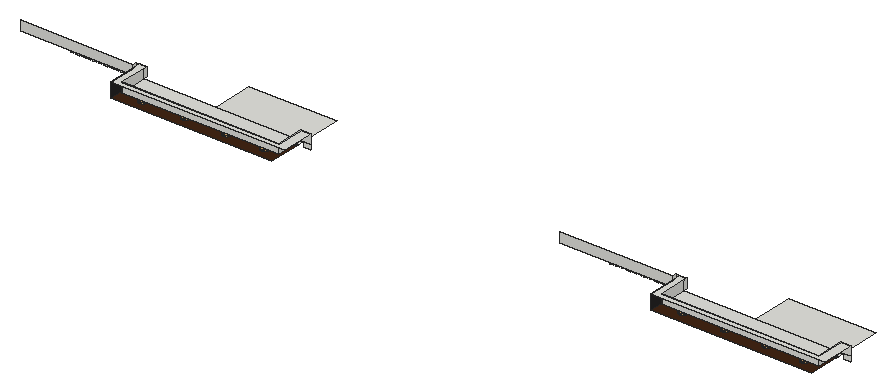
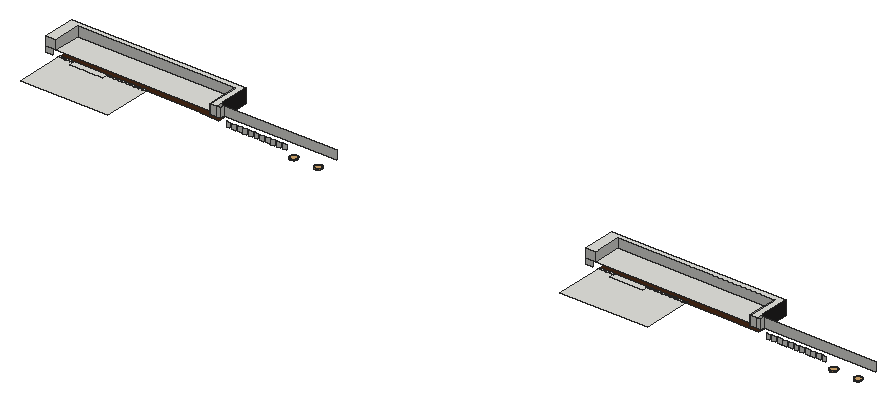
# SketchUp Ruby script. Lengths in inches.
U = 1.inch
M = Sketchup.active_model
def pt(a) = Geom::Point3d.new(a.map { |v| v * U })
def face(e, loops, mat)
  f = e.add_face(loops[0].map { |a| pt(a) })
  loops[1..].each { |l| e.add_face(l.map { |a| pt(a) }).erase! }
  f.material = f.back_material = mat if mat
  f
end
# faces: each face lists its corners as indices into pts; further lists are holes
def faces(e, pts, list, mat = nil) = list.each { |f| face(e, (f[0].is_a?(Array) ? f : [f]).map { |l| l.map { |i| pts[i] } }, mat) }
# xy, xz, yz: faces in a plane at the given z, y or x. An outline is a flat list of corners, or four numbers for a rectangle; further outlines are holes
def ring(l) = l.size == 4 ? [[l[0], l[1]], [l[2], l[1]], [l[2], l[3]], [l[0], l[3]]] : l.each_slice(2).to_a
def flat(e, list, mat, &to3) = list.each { |f| face(e, (f[0].is_a?(Array) ? f : [f]).map { |l| ring(l).map { |u, v| to3.(u, v) } }, mat) }
def xy(e, z, list, mat = nil) = flat(e, list, mat) { |x, y| [x, y, z] }
def xz(e, y, list, mat = nil) = flat(e, list, mat) { |x, z| [x, y, z] }
def yz(e, x, list, mat = nil) = flat(e, list, mat) { |y, z| [x, y, z] }
def lines(e, pts, list) = list.each { |a, b| e.add_line(pt(pts[a]), pt(pts[b])) }
# prism: a flat outline (further loops are holes) pulled along v
def prism(e, loops, v, mat = nil)
  f = face(e, loops, mat); d = Geom::Vector3d.new(v.map { |x| x * U })
  f.pushpull(f.normal.samedirection?(d) ? d.length : -d.length)
end
def box(e, o, s, mat = nil) = prism(e, [[o, [o[0] + s[0], o[1], o[2]], [o[0] + s[0], o[1] + s[1], o[2]], [o[0], o[1] + s[1], o[2]]]], [0, 0, s[2]], mat)
def at(x, y, z, deg = 0) = Geom::Transformation.translation(pt([x, y, z])) * Geom::Transformation.rotation(ORIGIN, Z_AXIS, deg.degrees)
def axes(o, x, y, z) = Geom::Transformation.new([*x, 0, *y, 0, *z, 0, *pt(o).to_a, 1])
def part(name) = M.definitions.add(name)
# library, detail: a bought-in or finely detailed component or shape, given as its bounding box
def library(name, o, s) = part(name).tap { |d| box(d.entities, o, s) }
def detail(e, o, s) = box(e.add_group.entities, o, s)
def put(e, d, t, mat = nil) = e.add_instance(d, t).tap { |i| i.material = mat if mat }
def group(e, t, mat = nil) = e.add_group.tap { |g| g.transformation = t; g.material = mat if mat }.entities
root = M.entities
M.materials.add("[Field Square Tile]").color = [211, 167, 108]
M.materials.add("[Granite Dark Gray]").color = [38, 37, 37]
M.materials.add("[Wood Veneer 01]").color = [66, 38, 20]
xy(root,380.5,[[534.46,508.33,539.88,511.08],[539.88,508.33,541.08,511.08],[541.08,508.33,546.51,511.08],[546.51,508.33,547.71,511.08],[547.71,508.33,553.13,511.08],
  [553.13,508.33,554.33,511.08],[554.33,508.33,559.76,511.08],[559.76,508.33,560.96,511.08],[560.96,508.33,566.38,511.08],[566.38,508.33,567.58,511.08],
  [567.58,508.33,573.01,511.08],[573.01,508.33,574.21,511.08],[574.21,508.33,579.63,511.08],[579.63,508.33,580.83,511.08],[580.83,508.33,586.26,511.08],
  [586.26,508.33,587.46,511.08],[587.46,508.33,592.88,511.08],[592.88,508.33,594.08,511.08],[594.08,508.33,599.51,511.08],[599.51,508.33,653.06,518.65],
  [653.06,508.33,658.48,511.08],[658.48,508.33,659.68,511.08],[659.68,508.33,665.11,511.08],[665.11,508.33,666.31,511.08],[666.31,508.33,671.73,511.08],
  [671.73,508.33,672.56,511.08],[672.56,508.33,676.54,511.08],[676.54,508.33,677.98,511.08],[1413.21,508.33,1418.63,511.08],[1418.63,508.33,1419.83,511.08],
  [1419.83,508.33,1425.26,511.08],[1425.26,508.33,1426.46,511.08],[1426.46,508.33,1431.88,511.08],[1431.88,508.33,1433.08,511.08],[1433.08,508.33,1438.51,511.08],
  [1438.51,508.33,1439.71,511.08],[1439.71,508.33,1445.13,511.08],[1445.13,508.33,1446.33,511.08],[1446.33,508.33,1451.76,511.08],[1451.76,508.33,1452.96,511.08],
  [1452.96,508.33,1458.38,511.08],[1458.38,508.33,1459.58,511.08],[1459.58,508.33,1465.01,511.08],[1465.01,508.33,1466.21,511.08],[1466.21,508.33,1471.63,511.08],
  [1471.63,508.33,1472.83,511.08],[1472.83,508.33,1478.26,511.08],[1478.26,508.33,1531.81,518.65],[1531.81,508.33,1537.23,511.08],[1537.23,508.33,1538.43,511.08],
  [1538.43,508.33,1543.86,511.08],[1543.86,508.33,1545.06,511.08],[1545.06,508.33,1550.48,511.08],[1550.48,508.33,1551.31,511.08],[1551.31,508.33,1555.29,511.08],
  [1555.29,508.33,1556.73,511.08],[534.46,511.08,534.46,589.83,676.54,589.83,676.54,511.08,653.06,511.08,653.06,518.65,599.51,518.65,599.51,511.08],[1413.21,511.08,1413.21,589.83,1555.29,589.83,1555.29,511.08,1531.81,511.08,1531.81,518.65,1478.26,518.65,1478.26,511.08]])
xy(root,380.5,[[[414.98,458.5,414.98,512.27,444.78,512.27,444.78,511.08,534.46,511.08,534.46,508.33,676.54,508.33,676.54,458.5],[521.68,470.7,523.23,470.9,524.68,471.5,525.92,472.46,526.88,473.7,527.48,475.15,527.68,476.7,527.48,478.25,526.88,479.7,525.92,480.94,524.68,481.9,523.23,482.49,521.68,482.7,520.13,482.49,518.68,481.9,517.4375,480.94,516.49,479.7,515.89,478.25,515.68,476.7,515.89,475.15,516.49,473.7,517.4375,472.46,518.68,471.5,520.13,470.9],[588.96,470.7,590.51,470.9,591.96,471.5,593.2,472.46,594.16,473.7,594.76,475.15,594.96,476.7,594.76,478.25,594.16,479.7,593.2,480.94,591.96,481.9,590.51,482.49,588.96,482.7,587.41,482.49,585.96,481.9,584.72,480.94,583.76,479.7,583.16,478.25,582.96,476.7,583.16,475.15,583.76,473.7,584.72,472.46,585.96,471.5,587.41,470.9],[650.33,470.7,651.89,470.9,653.33,471.5,654.58,472.46,655.53,473.7,656.13,475.15,656.33,476.7,656.13,478.25,655.53,479.7,654.58,480.94,653.33,481.9,651.89,482.49,650.33,482.7,648.78,482.49,647.33,481.9,646.09,480.94,645.14,479.7,644.54,478.25,644.33,476.7,644.54,475.15,645.14,473.7,646.09,472.46,647.33,471.5,648.78,470.9],[452.22,470.7,453.77,470.9,455.22,471.5,456.46,472.46,457.41,473.7,458.01,475.15,458.22,476.7,458.01,478.25,457.41,479.7,456.46,480.94,455.22,481.9,453.77,482.49,452.22,482.7,450.67,482.49,449.22,481.9,447.98,480.94,447.02,479.7,446.42,478.25,446.22,476.7,446.42,475.15,447.02,473.7,447.98,472.46,449.22,471.5,450.67,470.9]],[[1293.73,458.5,1293.73,512.27,1323.53,512.27,1323.53,511.08,1413.21,511.08,1413.21,508.33,1555.29,508.33,1555.29,458.5],[1400.43,470.7,1401.98,470.9,1403.43,471.5,1404.67,472.46,1405.63,473.7,1406.23,475.15,1406.43,476.7,1406.23,478.25,1405.63,479.7,1404.67,480.94,1403.43,481.9,1401.98,482.49,1400.43,482.7,1398.88,482.49,1397.43,481.9,1396.1875,480.94,1395.24,479.7,1394.64,478.25,1394.43,476.7,1394.64,475.15,1395.24,473.7,1396.1875,472.46,1397.43,471.5,1398.88,470.9],[1529.08,470.7,1530.64,470.9,1532.08,471.5,1533.33,472.46,1534.28,473.7,1534.88,475.15,1535.08,476.7,1534.88,478.25,1534.28,479.7,1533.33,480.94,1532.08,481.9,1530.64,482.49,1529.08,482.7,1527.53,482.49,1526.08,481.9,1524.84,480.94,1523.89,479.7,1523.29,478.25,1523.08,476.7,1523.29,475.15,1523.89,473.7,1524.84,472.46,1526.08,471.5,1527.53,470.9],[1330.97,470.7,1332.52,470.9,1333.97,471.5,1335.21,472.46,1336.16,473.7,1336.76,475.15,1336.97,476.7,1336.76,478.25,1336.16,479.7,1335.21,480.94,1333.97,481.9,1332.52,482.49,1330.97,482.7,1329.42,482.49,1327.97,481.9,1326.73,480.94,1325.77,479.7,1325.17,478.25,1324.97,476.7,1325.17,475.15,1325.77,473.7,1326.73,472.46,1327.97,471.5,1329.42,470.9],[1467.71,470.7,1469.26,470.9,1470.71,471.5,1471.95,472.46,1472.91,473.7,1473.51,475.15,1473.71,476.7,1473.51,478.25,1472.91,479.7,1471.95,480.94,1470.71,481.9,1469.26,482.49,1467.71,482.7,1466.16,482.49,1464.71,481.9,1463.47,480.94,1462.51,479.7,1461.91,478.25,1461.71,476.7,1461.91,475.15,1462.51,473.7,1463.47,472.46,1464.71,471.5,1466.16,470.9]]],"[Wood Veneer 01]")
xy(root,381.8125,[[452.22,470.7,450.67,470.9,449.22,471.5,447.98,472.46,447.02,473.7,446.42,475.15,446.22,476.7,446.42,478.25,447.02,479.7,447.98,480.94,449.22,481.9,450.67,482.49,452.22,482.7,453.77,482.49,455.22,481.9,456.46,480.94,457.41,479.7,458.01,478.25,458.22,476.7,458.01,475.15,457.41,473.7,456.46,472.46,455.22,471.5,453.77,470.9],[521.68,470.7,520.13,470.9,518.68,471.5,517.4375,472.46,516.49,473.7,515.89,475.15,515.68,476.7,515.89,478.25,516.49,479.7,517.4375,480.94,518.68,481.9,520.13,482.49,521.68,482.7,523.23,482.49,524.68,481.9,525.92,480.94,526.88,479.7,527.48,478.25,527.68,476.7,527.48,475.15,526.88,473.7,525.92,472.46,524.68,471.5,523.23,470.9],[588.96,470.7,587.41,470.9,585.96,471.5,584.72,472.46,583.76,473.7,583.16,475.15,582.96,476.7,583.16,478.25,583.76,479.7,584.72,480.94,585.96,481.9,587.41,482.49,588.96,482.7,590.51,482.49,591.96,481.9,593.2,480.94,594.16,479.7,594.76,478.25,594.96,476.7,594.76,475.15,594.16,473.7,593.2,472.46,591.96,471.5,590.51,470.9],[650.33,470.7,648.78,470.9,647.33,471.5,646.09,472.46,645.14,473.7,644.54,475.15,644.33,476.7,644.54,478.25,645.14,479.7,646.09,480.94,647.33,481.9,648.78,482.49,650.33,482.7,651.89,482.49,653.33,481.9,654.58,480.94,655.53,479.7,656.13,478.25,656.33,476.7,656.13,475.15,655.53,473.7,654.58,472.46,653.33,471.5,651.89,470.9],[1330.97,470.7,1329.42,470.9,1327.97,471.5,1326.73,472.46,1325.77,473.7,1325.17,475.15,1324.97,476.7,1325.17,478.25,1325.77,479.7,1326.73,480.94,1327.97,481.9,1329.42,482.49,1330.97,482.7,1332.52,482.49,1333.97,481.9,1335.21,480.94,1336.16,479.7,1336.76,478.25,1336.97,476.7,1336.76,475.15,1336.16,473.7,1335.21,472.46,1333.97,471.5,1332.52,470.9],
  [1400.43,470.7,1398.88,470.9,1397.43,471.5,1396.1875,472.46,1395.24,473.7,1394.64,475.15,1394.43,476.7,1394.64,478.25,1395.24,479.7,1396.1875,480.94,1397.43,481.9,1398.88,482.49,1400.43,482.7,1401.98,482.49,1403.43,481.9,1404.67,480.94,1405.63,479.7,1406.23,478.25,1406.43,476.7,1406.23,475.15,1405.63,473.7,1404.67,472.46,1403.43,471.5,1401.98,470.9],[1467.71,470.7,1466.16,470.9,1464.71,471.5,1463.47,472.46,1462.51,473.7,1461.91,475.15,1461.71,476.7,1461.91,478.25,1462.51,479.7,1463.47,480.94,1464.71,481.9,1466.16,482.49,1467.71,482.7,1469.26,482.49,1470.71,481.9,1471.95,480.94,1472.91,479.7,1473.51,478.25,1473.71,476.7,1473.51,475.15,1472.91,473.7,1471.95,472.46,1470.71,471.5,1469.26,470.9],[1529.08,470.7,1527.53,470.9,1526.08,471.5,1524.84,472.46,1523.89,473.7,1523.29,475.15,1523.08,476.7,1523.29,478.25,1523.89,479.7,1524.84,480.94,1526.08,481.9,1527.53,482.49,1529.08,482.7,1530.64,482.49,1532.08,481.9,1533.33,480.94,1534.28,479.7,1534.88,478.25,1535.08,476.7,1534.88,475.15,1534.28,473.7,1533.33,472.46,1532.08,471.5,1530.64,470.9]],"[Field Square Tile]")
xy(root,381.875,[[240.83,523.51,239.27,523.54,237.76,523.98,236.42,524.79,235.34,525.92,234.58,527.29,234.21,528.8125,234.24,530.375,234.68,531.88,235.49,533.22,236.62,534.31,237.99,535.06,239.51,535.43,241.08,535.4,242.58,534.96,243.92,534.15,245.01,533.02,245.76,531.65,246.14,530.13,246.1,528.5625,245.67,527.06,244.86,525.72,243.73,524.64,242.35,523.88],[280.58,523.51,279.02,523.54,277.51,523.98,276.17,524.79,275.09,525.92,274.33,527.29,273.96,528.8125,273.99,530.375,274.43,531.88,275.24,533.22,276.37,534.31,277.74,535.06,279.26,535.43,280.83,535.4,282.33,534.96,283.67,534.15,284.76,533.02,285.51,531.65,285.89,530.13,285.85,528.5625,285.42,527.06,284.61,525.72,283.48,524.64,282.1,523.88],[1119.58,523.51,1118.02,523.54,1116.51,523.98,1115.17,524.79,1114.09,525.92,1113.33,527.29,1112.96,528.8125,1112.99,530.375,1113.43,531.88,1114.24,533.22,1115.37,534.31,1116.74,535.06,1118.26,535.43,1119.83,535.4,1121.33,534.96,1122.67,534.15,1123.76,533.02,1124.51,531.65,1124.89,530.13,1124.85,528.5625,1124.42,527.06,1123.61,525.72,1122.48,524.64,1121.1,523.88],[1159.33,523.51,1157.77,523.54,1156.26,523.98,1154.92,524.79,1153.84,525.92,1153.08,527.29,1152.71,528.8125,1152.74,530.375,1153.18,531.88,1153.99,533.22,1155.12,534.31,1156.49,535.06,1158.01,535.43,1159.58,535.4,1161.08,534.96,1162.42,534.15,1163.51,533.02,1164.26,531.65,1164.64,530.13,1164.6,528.5625,1164.17,527.06,1163.36,525.72,1162.23,524.64,1160.85,523.88]],"[Field Square Tile]")
xy(root,388.625,[[425.6875,466.05,682.18,511.08],[1304.4375,466.05,1560.93,511.08]])
xy(root,403.8125,[[414.98,458.5,698.16,458.5,698.16,511.08,682.18,511.08,682.18,466.05,425.6875,466.05,425.6875,517.43,414.98,517.43],[1293.73,458.5,1576.91,458.5,1576.91,511.08,1560.93,511.08,1560.93,466.05,1304.4375,466.05,1304.4375,517.43,1293.73,517.43]])
xz(root,466.05,[[425.6875,388.625,682.18,403.8125],[1304.4375,388.625,1560.93,403.8125]])
xz(root,510.87,[[225.31,388.625,408.63,403.8125],[1104.06,388.625,1287.38,403.8125]])
xz(root,511.08,[[686.35,380.5,698.16,388.625],[1565.1,380.5,1576.91,388.625],[682.18,388.625,698.16,403.8125],[1560.93,388.625,1576.91,403.8125]])
xz(root,517.43,[[408.63,388.625,414.98,403.8125],[414.98,388.625,425.6875,403.8125],[1287.38,388.625,1293.73,403.8125],[1293.73,388.625,1304.4375,403.8125]])
xz(root,519.43,[[299.93,380.5,306.18,388.625],[309.06,380.5,315.31,388.625],[318.18,380.5,324.43,388.625],[327.31,380.5,333.56,388.625],[336.43,380.5,342.68,388.625],
  [345.56,380.5,351.81,388.625],[354.68,380.5,360.93,388.625],[363.81,380.5,370.06,388.625],[372.93,380.5,379.18,388.625],[382.06,380.5,388.31,388.625],
  [391.18,380.5,397.43,388.625],[1178.68,380.5,1184.93,388.625],[1187.81,380.5,1194.06,388.625],[1196.93,380.5,1203.18,388.625],[1206.06,380.5,1212.31,388.625],
  [1215.18,380.5,1221.43,388.625],[1224.31,380.5,1230.56,388.625],[1233.43,380.5,1239.68,388.625],[1242.56,380.5,1248.81,388.625],[1251.68,380.5,1257.93,388.625],
  [1260.81,380.5,1267.06,388.625],[1269.93,380.5,1276.18,388.625]])
yz(root,408.63,[[510.87,388.625,517.43,403.8125]])
yz(root,414.98,[[458.5,380.5,504.52,403.8125]],"[Granite Dark Gray]")
yz(root,425.6875,[[466.05,388.625,511.08,403.8125],[511.08,388.625,517.43,403.8125]])
yz(root,682.18,[[466.05,388.625,511.08,403.8125]])
yz(root,1287.38,[[510.87,388.625,517.43,403.8125]])
yz(root,1293.73,[[458.5,380.5,504.52,403.8125]],"[Granite Dark Gray]")
yz(root,1304.4375,[[466.05,388.625,511.08,403.8125],[511.08,388.625,517.43,403.8125]])
yz(root,1560.93,[[466.05,388.625,511.08,403.8125]])
p = [[452.22,470.7,380.5],[450.67,470.9,380.5],[450.67,470.9,381.8125],[452.22,470.7,381.8125],[453.77,470.9,380.5],[453.77,470.9,381.8125],
  [521.68,470.7,380.5],[520.13,470.9,380.5],[520.13,470.9,381.8125],[521.68,470.7,381.8125],[523.23,470.9,380.5],[523.23,470.9,381.8125],
  [588.96,470.7,380.5],[587.41,470.9,380.5],[587.41,470.9,381.8125],[588.96,470.7,381.8125],[590.51,470.9,380.5],[590.51,470.9,381.8125],
  [650.33,470.7,380.5],[648.78,470.9,380.5],[648.78,470.9,381.8125],[650.33,470.7,381.8125],[651.89,470.9,380.5],[651.89,470.9,381.8125],
  [1330.97,470.7,380.5],[1329.42,470.9,380.5],[1329.42,470.9,381.8125],[1330.97,470.7,381.8125],[1332.52,470.9,380.5],[1332.52,470.9,381.8125],
  [1400.43,470.7,380.5],[1398.88,470.9,380.5],[1398.88,470.9,381.8125],[1400.43,470.7,381.8125],[1401.98,470.9,380.5],[1401.98,470.9,381.8125],
  [1467.71,470.7,380.5],[1466.16,470.9,380.5],[1466.16,470.9,381.8125],[1467.71,470.7,381.8125],[1469.26,470.9,380.5],[1469.26,470.9,381.8125],
  [1529.08,470.7,380.5],[1527.53,470.9,380.5],[1527.53,470.9,381.8125],[1529.08,470.7,381.8125],[1530.64,470.9,380.5],[1530.64,470.9,381.8125],
  [449.22,471.5,380.5],[449.22,471.5,381.8125],[455.22,471.5,380.5],[455.22,471.5,381.8125],[518.68,471.5,380.5],[518.68,471.5,381.8125],
  [524.68,471.5,380.5],[524.68,471.5,381.8125],[585.96,471.5,380.5],[585.96,471.5,381.8125],[591.96,471.5,380.5],[591.96,471.5,381.8125],
  [647.33,471.5,380.5],[647.33,471.5,381.8125],[653.33,471.5,380.5],[653.33,471.5,381.8125],[1327.97,471.5,380.5],[1327.97,471.5,381.8125],
  [1333.97,471.5,380.5],[1333.97,471.5,381.8125],[1397.43,471.5,380.5],[1397.43,471.5,381.8125],[1403.43,471.5,380.5],[1403.43,471.5,381.8125],
  [1464.71,471.5,380.5],[1464.71,471.5,381.8125],[1470.71,471.5,380.5],[1470.71,471.5,381.8125],[1526.08,471.5,380.5],[1526.08,471.5,381.8125],
  [1532.08,471.5,380.5],[1532.08,471.5,381.8125],[447.98,472.46,380.5],[447.98,472.46,381.8125],[456.46,472.46,380.5],[456.46,472.46,381.8125],
  [517.4375,472.46,380.5],[517.4375,472.46,381.8125],[525.92,472.46,380.5],[525.92,472.46,381.8125],[584.72,472.46,380.5],[584.72,472.46,381.8125],
  [593.2,472.46,380.5],[593.2,472.46,381.8125],[646.09,472.46,380.5],[646.09,472.46,381.8125],[654.58,472.46,380.5],[654.58,472.46,381.8125],
  [1326.73,472.46,380.5],[1326.73,472.46,381.8125],[1335.21,472.46,380.5],[1335.21,472.46,381.8125],[1396.1875,472.46,380.5],[1396.1875,472.46,381.8125],
  [1404.67,472.46,380.5],[1404.67,472.46,381.8125],[1463.47,472.46,380.5],[1463.47,472.46,381.8125],[1471.95,472.46,380.5],[1471.95,472.46,381.8125],
  [1524.84,472.46,380.5],[1524.84,472.46,381.8125],[1533.33,472.46,380.5],[1533.33,472.46,381.8125],[447.02,473.7,380.5],[447.02,473.7,381.8125],
  [457.41,473.7,380.5],[457.41,473.7,381.8125],[516.49,473.7,380.5],[516.49,473.7,381.8125],[526.88,473.7,380.5],[526.88,473.7,381.8125],
  [583.76,473.7,380.5],[583.76,473.7,381.8125],[594.16,473.7,380.5],[594.16,473.7,381.8125],[645.14,473.7,380.5],[645.14,473.7,381.8125],
  [655.53,473.7,380.5],[655.53,473.7,381.8125],[1325.77,473.7,380.5],[1325.77,473.7,381.8125],[1336.16,473.7,380.5],[1336.16,473.7,381.8125],
  [1395.24,473.7,380.5],[1395.24,473.7,381.8125],[1405.63,473.7,380.5],[1405.63,473.7,381.8125],[1462.51,473.7,380.5],[1462.51,473.7,381.8125],
  [1472.91,473.7,380.5],[1472.91,473.7,381.8125],[1523.89,473.7,380.5],[1523.89,473.7,381.8125],[1534.28,473.7,380.5],[1534.28,473.7,381.8125],
  [446.42,475.15,380.5],[446.42,475.15,381.8125],[458.01,475.15,380.5],[458.01,475.15,381.8125],[515.89,475.15,380.5],[515.89,475.15,381.8125],
  [527.48,475.15,380.5],[527.48,475.15,381.8125],[583.16,475.15,380.5],[583.16,475.15,381.8125],[594.76,475.15,380.5],[594.76,475.15,381.8125],
  [644.54,475.15,380.5],[644.54,475.15,381.8125],[656.13,475.15,380.5],[656.13,475.15,381.8125],[1325.17,475.15,380.5],[1325.17,475.15,381.8125],
  [1336.76,475.15,380.5],[1336.76,475.15,381.8125],[1394.64,475.15,380.5],[1394.64,475.15,381.8125],[1406.23,475.15,380.5],[1406.23,475.15,381.8125],
  [1461.91,475.15,380.5],[1461.91,475.15,381.8125],[1473.51,475.15,380.5],[1473.51,475.15,381.8125],[1523.29,475.15,380.5],[1523.29,475.15,381.8125],
  [1534.88,475.15,380.5],[1534.88,475.15,381.8125],[446.22,476.7,380.5],[446.22,476.7,381.8125],[458.22,476.7,380.5],[458.22,476.7,381.8125],
  [515.68,476.7,380.5],[515.68,476.7,381.8125],[527.68,476.7,380.5],[527.68,476.7,381.8125],[582.96,476.7,380.5],[582.96,476.7,381.8125],
  [594.96,476.7,380.5],[594.96,476.7,381.8125],[644.33,476.7,380.5],[644.33,476.7,381.8125],[656.33,476.7,380.5],[656.33,476.7,381.8125],
  [1324.97,476.7,380.5],[1324.97,476.7,381.8125],[1336.97,476.7,380.5],[1336.97,476.7,381.8125],[1394.43,476.7,380.5],[1394.43,476.7,381.8125],
  [1406.43,476.7,380.5],[1406.43,476.7,381.8125],[1461.71,476.7,380.5],[1461.71,476.7,381.8125],[1473.71,476.7,380.5],[1473.71,476.7,381.8125],
  [1523.08,476.7,380.5],[1523.08,476.7,381.8125],[1535.08,476.7,380.5],[1535.08,476.7,381.8125],[446.42,478.25,380.5],[446.42,478.25,381.8125],
  [458.01,478.25,380.5],[458.01,478.25,381.8125],[515.89,478.25,380.5],[515.89,478.25,381.8125],[527.48,478.25,380.5],[527.48,478.25,381.8125],
  [583.16,478.25,380.5],[583.16,478.25,381.8125],[594.76,478.25,380.5],[594.76,478.25,381.8125],[644.54,478.25,380.5],[644.54,478.25,381.8125],
  [656.13,478.25,380.5],[656.13,478.25,381.8125],[1325.17,478.25,380.5],[1325.17,478.25,381.8125],[1336.76,478.25,380.5],[1336.76,478.25,381.8125],
  [1394.64,478.25,380.5],[1394.64,478.25,381.8125],[1406.23,478.25,380.5],[1406.23,478.25,381.8125],[1461.91,478.25,380.5],[1461.91,478.25,381.8125],
  [1473.51,478.25,380.5],[1473.51,478.25,381.8125],[1523.29,478.25,380.5],[1523.29,478.25,381.8125],[1534.88,478.25,380.5],[1534.88,478.25,381.8125],
  [447.02,479.7,380.5],[447.02,479.7,381.8125],[457.41,479.7,380.5],[457.41,479.7,381.8125],[516.49,479.7,380.5],[516.49,479.7,381.8125],
  [526.88,479.7,380.5],[526.88,479.7,381.8125],[583.76,479.7,380.5],[583.76,479.7,381.8125],[594.16,479.7,380.5],[594.16,479.7,381.8125],
  [645.14,479.7,380.5],[645.14,479.7,381.8125],[655.53,479.7,380.5],[655.53,479.7,381.8125],[1325.77,479.7,380.5],[1325.77,479.7,381.8125],
  [1336.16,479.7,380.5],[1336.16,479.7,381.8125],[1395.24,479.7,380.5],[1395.24,479.7,381.8125],[1405.63,479.7,380.5],[1405.63,479.7,381.8125],
  [1462.51,479.7,380.5],[1462.51,479.7,381.8125],[1472.91,479.7,380.5],[1472.91,479.7,381.8125],[1523.89,479.7,380.5],[1523.89,479.7,381.8125],
  [1534.28,479.7,380.5],[1534.28,479.7,381.8125],[447.98,480.94,380.5],[447.98,480.94,381.8125],[456.46,480.94,380.5],[456.46,480.94,381.8125],
  [517.4375,480.94,380.5],[517.4375,480.94,381.8125],[525.92,480.94,380.5],[525.92,480.94,381.8125],[584.72,480.94,380.5],[584.72,480.94,381.8125],
  [593.2,480.94,380.5],[593.2,480.94,381.8125],[646.09,480.94,380.5],[646.09,480.94,381.8125],[654.58,480.94,380.5],[654.58,480.94,381.8125],
  [1326.73,480.94,380.5],[1326.73,480.94,381.8125],[1335.21,480.94,380.5],[1335.21,480.94,381.8125],[1396.1875,480.94,380.5],[1396.1875,480.94,381.8125],
  [1404.67,480.94,380.5],[1404.67,480.94,381.8125],[1463.47,480.94,380.5],[1463.47,480.94,381.8125],[1471.95,480.94,380.5],[1471.95,480.94,381.8125],
  [1524.84,480.94,380.5],[1524.84,480.94,381.8125],[1533.33,480.94,380.5],[1533.33,480.94,381.8125],[449.22,481.9,380.5],[449.22,481.9,381.8125],
  [455.22,481.9,380.5],[455.22,481.9,381.8125],[518.68,481.9,380.5],[518.68,481.9,381.8125],[524.68,481.9,380.5],[524.68,481.9,381.8125],
  [585.96,481.9,380.5],[585.96,481.9,381.8125],[591.96,481.9,380.5],[591.96,481.9,381.8125],[647.33,481.9,380.5],[647.33,481.9,381.8125],
  [653.33,481.9,380.5],[653.33,481.9,381.8125],[1327.97,481.9,380.5],[1327.97,481.9,381.8125],[1333.97,481.9,380.5],[1333.97,481.9,381.8125],
  [1397.43,481.9,380.5],[1397.43,481.9,381.8125],[1403.43,481.9,380.5],[1403.43,481.9,381.8125],[1464.71,481.9,380.5],[1464.71,481.9,381.8125],
  [1470.71,481.9,380.5],[1470.71,481.9,381.8125],[1526.08,481.9,380.5],[1526.08,481.9,381.8125],[1532.08,481.9,380.5],[1532.08,481.9,381.8125],
  [450.67,482.49,380.5],[450.67,482.49,381.8125],[453.77,482.49,380.5],[453.77,482.49,381.8125],[520.13,482.49,380.5],[520.13,482.49,381.8125],
  [523.23,482.49,380.5],[523.23,482.49,381.8125],[587.41,482.49,380.5],[587.41,482.49,381.8125],[590.51,482.49,380.5],[590.51,482.49,381.8125],
  [648.78,482.49,380.5],[648.78,482.49,381.8125],[651.89,482.49,380.5],[651.89,482.49,381.8125],[1329.42,482.49,380.5],[1329.42,482.49,381.8125],
  [1332.52,482.49,380.5],[1332.52,482.49,381.8125],[1398.88,482.49,380.5],[1398.88,482.49,381.8125],[1401.98,482.49,380.5],[1401.98,482.49,381.8125],
  [1466.16,482.49,380.5],[1466.16,482.49,381.8125],[1469.26,482.49,380.5],[1469.26,482.49,381.8125],[1527.53,482.49,380.5],[1527.53,482.49,381.8125],
  [1530.64,482.49,380.5],[1530.64,482.49,381.8125],[452.22,482.7,380.5],[452.22,482.7,381.8125],[521.68,482.7,380.5],[521.68,482.7,381.8125],
  [588.96,482.7,380.5],[588.96,482.7,381.8125],[650.33,482.7,380.5],[650.33,482.7,381.8125],[1330.97,482.7,380.5],[1330.97,482.7,381.8125],
  [1400.43,482.7,380.5],[1400.43,482.7,381.8125],[1467.71,482.7,380.5],[1467.71,482.7,381.8125],[1529.08,482.7,380.5],[1529.08,482.7,381.8125],
  [239.27,523.54,380.5],[237.76,523.98,380.5],[237.76,523.98,381.875],[239.27,523.54,381.875],[240.83,523.51,380.5],[240.83,523.51,381.875],
  [242.35,523.88,380.5],[242.35,523.88,381.875],[279.02,523.54,380.5],[277.51,523.98,380.5],[277.51,523.98,381.875],[279.02,523.54,381.875],
  [280.58,523.51,380.5],[280.58,523.51,381.875],[282.1,523.88,380.5],[282.1,523.88,381.875],[1118.02,523.54,380.5],[1116.51,523.98,380.5],
  [1116.51,523.98,381.875],[1118.02,523.54,381.875],[1119.58,523.51,380.5],[1119.58,523.51,381.875],[1121.1,523.88,380.5],[1121.1,523.88,381.875],
  [1157.77,523.54,380.5],[1156.26,523.98,380.5],[1156.26,523.98,381.875],[1157.77,523.54,381.875],[1159.33,523.51,380.5],[1159.33,523.51,381.875],
  [1160.85,523.88,380.5],[1160.85,523.88,381.875],[243.73,524.64,380.5],[243.73,524.64,381.875],[283.48,524.64,380.5],[283.48,524.64,381.875],
  [1122.48,524.64,380.5],[1122.48,524.64,381.875],[1162.23,524.64,380.5],[1162.23,524.64,381.875],[236.42,524.79,380.5],[236.42,524.79,381.875],
  [276.17,524.79,380.5],[276.17,524.79,381.875],[1115.17,524.79,380.5],[1115.17,524.79,381.875],[1154.92,524.79,380.5],[1154.92,524.79,381.875],
  [244.86,525.72,380.5],[244.86,525.72,381.875],[284.61,525.72,380.5],[284.61,525.72,381.875],[1123.61,525.72,380.5],[1123.61,525.72,381.875],
  [1163.36,525.72,380.5],[1163.36,525.72,381.875],[235.34,525.92,380.5],[235.34,525.92,381.875],[275.09,525.92,380.5],[275.09,525.92,381.875],
  [1114.09,525.92,380.5],[1114.09,525.92,381.875],[1153.84,525.92,380.5],[1153.84,525.92,381.875],[245.67,527.06,380.5],[245.67,527.06,381.875],
  [285.42,527.06,380.5],[285.42,527.06,381.875],[1124.42,527.06,380.5],[1124.42,527.06,381.875],[1164.17,527.06,380.5],[1164.17,527.06,381.875],
  [234.58,527.29,380.5],[234.58,527.29,381.875],[274.33,527.29,380.5],[274.33,527.29,381.875],[1113.33,527.29,380.5],[1113.33,527.29,381.875],
  [1153.08,527.29,380.5],[1153.08,527.29,381.875],[246.1,528.5625,380.5],[246.1,528.5625,381.875],[285.85,528.5625,380.5],[285.85,528.5625,381.875],
  [1124.85,528.5625,380.5],[1124.85,528.5625,381.875],[1164.6,528.5625,380.5],[1164.6,528.5625,381.875],[234.21,528.8125,380.5],[234.21,528.8125,381.875],
  [273.96,528.8125,380.5],[273.96,528.8125,381.875],[1112.96,528.8125,380.5],[1112.96,528.8125,381.875],[1152.71,528.8125,380.5],[1152.71,528.8125,381.875],
  [246.14,530.13,380.5],[246.14,530.13,381.875],[285.89,530.13,380.5],[285.89,530.13,381.875],[1124.89,530.13,380.5],[1124.89,530.13,381.875],
  [1164.64,530.13,380.5],[1164.64,530.13,381.875],[234.24,530.375,380.5],[234.24,530.375,381.875],[273.99,530.375,380.5],[273.99,530.375,381.875],
  [1112.99,530.375,380.5],[1112.99,530.375,381.875],[1152.74,530.375,380.5],[1152.74,530.375,381.875],[245.76,531.65,380.5],[245.76,531.65,381.875],
  [285.51,531.65,380.5],[285.51,531.65,381.875],[1124.51,531.65,380.5],[1124.51,531.65,381.875],[1164.26,531.65,380.5],[1164.26,531.65,381.875],
  [234.68,531.88,380.5],[234.68,531.88,381.875],[274.43,531.88,380.5],[274.43,531.88,381.875],[1113.43,531.88,380.5],[1113.43,531.88,381.875],
  [1153.18,531.88,380.5],[1153.18,531.88,381.875],[245.01,533.02,380.5],[245.01,533.02,381.875],[284.76,533.02,380.5],[284.76,533.02,381.875],
  [1123.76,533.02,380.5],[1123.76,533.02,381.875],[1163.51,533.02,380.5],[1163.51,533.02,381.875],[235.49,533.22,380.5],[235.49,533.22,381.875],
  [275.24,533.22,380.5],[275.24,533.22,381.875],[1114.24,533.22,380.5],[1114.24,533.22,381.875],[1153.99,533.22,380.5],[1153.99,533.22,381.875],
  [243.92,534.15,380.5],[243.92,534.15,381.875],[283.67,534.15,380.5],[283.67,534.15,381.875],[1122.67,534.15,380.5],[1122.67,534.15,381.875],
  [1162.42,534.15,380.5],[1162.42,534.15,381.875],[236.62,534.31,380.5],[236.62,534.31,381.875],[276.37,534.31,380.5],[276.37,534.31,381.875],
  [1115.37,534.31,380.5],[1115.37,534.31,381.875],[1155.12,534.31,380.5],[1155.12,534.31,381.875],[242.58,534.96,380.5],[242.58,534.96,381.875],
  [282.33,534.96,380.5],[282.33,534.96,381.875],[1121.33,534.96,380.5],[1121.33,534.96,381.875],[1161.08,534.96,380.5],[1161.08,534.96,381.875],
  [237.99,535.06,380.5],[237.99,535.06,381.875],[277.74,535.06,380.5],[277.74,535.06,381.875],[1116.74,535.06,380.5],[1116.74,535.06,381.875],
  [1156.49,535.06,380.5],[1156.49,535.06,381.875],[241.08,535.4,380.5],[241.08,535.4,381.875],[280.83,535.4,380.5],[280.83,535.4,381.875],
  [1119.83,535.4,380.5],[1119.83,535.4,381.875],[1159.58,535.4,380.5],[1159.58,535.4,381.875],[239.51,535.43,380.5],[239.51,535.43,381.875],
  [279.26,535.43,380.5],[279.26,535.43,381.875],[1118.26,535.43,380.5],[1118.26,535.43,381.875],[1158.01,535.43,380.5],[1158.01,535.43,381.875],
  [415,468.31,380.5],[414.98,458.5,380.5],[1293.75,468.31,380.5],[1293.73,458.5,380.5]]
faces(root,p,[[0,1,2,3],[4,0,3,5],[6,7,8,9],[10,6,9,11],[12,13,14,15],[16,12,15,17],[18,19,20,21],[22,18,21,23],
  [24,25,26,27],[28,24,27,29],[30,31,32,33],[34,30,33,35],[36,37,38,39],[40,36,39,41],[42,43,44,45],[46,42,45,47],
  [1,48,49,2],[50,4,5,51],[7,52,53,8],[54,10,11,55],[13,56,57,14],[58,16,17,59],[19,60,61,20],[62,22,23,63],
  [25,64,65,26],[66,28,29,67],[31,68,69,32],[70,34,35,71],[37,72,73,38],[74,40,41,75],[43,76,77,44],[78,46,47,79],
  [48,80,81,49],[82,50,51,83],[52,84,85,53],[86,54,55,87],[56,88,89,57],[90,58,59,91],[60,92,93,61],[94,62,63,95],
  [64,96,97,65],[98,66,67,99],[68,100,101,69],[102,70,71,103],[72,104,105,73],[106,74,75,107],[76,108,109,77],[110,78,79,111],
  [80,112,113,81],[114,82,83,115],[84,116,117,85],[118,86,87,119],[88,120,121,89],[122,90,91,123],[92,124,125,93],[126,94,95,127],
  [96,128,129,97],[130,98,99,131],[100,132,133,101],[134,102,103,135],[104,136,137,105],[138,106,107,139],[108,140,141,109],[142,110,111,143],
  [112,144,145,113],[146,114,115,147],[116,148,149,117],[150,118,119,151],[120,152,153,121],[154,122,123,155],[124,156,157,125],[158,126,127,159],
  [128,160,161,129],[162,130,131,163],[132,164,165,133],[166,134,135,167],[136,168,169,137],[170,138,139,171],[140,172,173,141],[174,142,143,175],
  [144,176,177,145],[178,146,147,179],[148,180,181,149],[182,150,151,183],[152,184,185,153],[186,154,155,187],[156,188,189,157],[190,158,159,191],
  [160,192,193,161],[194,162,163,195],[164,196,197,165],[198,166,167,199],[168,200,201,169],[202,170,171,203],[172,204,205,173],[206,174,175,207],
  [176,208,209,177],[210,178,179,211],[180,212,213,181],[214,182,183,215],[184,216,217,185],[218,186,187,219],[188,220,221,189],[222,190,191,223],
  [192,224,225,193],[226,194,195,227],[196,228,229,197],[230,198,199,231],[200,232,233,201],[234,202,203,235],[204,236,237,205],[238,206,207,239],
  [208,240,241,209],[242,210,211,243],[212,244,245,213],[246,214,215,247],[216,248,249,217],[250,218,219,251],[220,252,253,221],[254,222,223,255],
  [224,256,257,225],[258,226,227,259],[228,260,261,229],[262,230,231,263],[232,264,265,233],[266,234,235,267],[236,268,269,237],[270,238,239,271],
  [240,272,273,241],[274,242,243,275],[244,276,277,245],[278,246,247,279],[248,280,281,249],[282,250,251,283],[252,284,285,253],[286,254,255,287],
  [256,288,289,257],[290,258,259,291],[260,292,293,261],[294,262,263,295],[264,296,297,265],[298,266,267,299],[268,300,301,269],[302,270,271,303],
  [272,304,305,273],[306,274,275,307],[276,308,309,277],[310,278,279,311],[280,312,313,281],[314,282,283,315],[284,316,317,285],[318,286,287,319],
  [288,320,321,289],[322,290,291,323],[292,324,325,293],[326,294,295,327],[296,328,329,297],[330,298,299,331],[300,332,333,301],[334,302,303,335],
  [304,336,337,305],[338,306,307,339],[308,340,341,309],[342,310,311,343],[312,344,345,313],[346,314,315,347],[316,348,349,317],[350,318,319,351],
  [320,352,353,321],[354,322,323,355],[324,356,357,325],[358,326,327,359],[328,360,361,329],[362,330,331,363],[332,364,365,333],[366,334,335,367],
  [336,368,369,337],[368,338,339,369],[340,370,371,341],[370,342,343,371],[344,372,373,345],[372,346,347,373],[348,374,375,349],[374,350,351,375],
  [352,376,377,353],[376,354,355,377],[356,378,379,357],[378,358,359,379],[360,380,381,361],[380,362,363,381],[364,382,383,365],[382,366,367,383],
  [384,385,386,387],[388,384,387,389],[390,388,389,391],[392,393,394,395],[396,392,395,397],[398,396,397,399],[400,401,402,403],[404,400,403,405],
  [406,404,405,407],[408,409,410,411],[412,408,411,413],[414,412,413,415],[416,390,391,417],[418,398,399,419],[420,406,407,421],[422,414,415,423],
  [385,424,425,386],[393,426,427,394],[401,428,429,402],[409,430,431,410],[432,416,417,433],[434,418,419,435],[436,420,421,437],[438,422,423,439],
  [424,440,441,425],[426,442,443,427],[428,444,445,429],[430,446,447,431],[448,432,433,449],[450,434,435,451],[452,436,437,453],[454,438,439,455],
  [440,456,457,441],[442,458,459,443],[444,460,461,445],[446,462,463,447],[464,448,449,465],[466,450,451,467],[468,452,453,469],[470,454,455,471],
  [456,472,473,457],[458,474,475,459],[460,476,477,461],[462,478,479,463],[480,464,465,481],[482,466,467,483],[484,468,469,485],[486,470,471,487],
  [472,488,489,473],[474,490,491,475],[476,492,493,477],[478,494,495,479],[496,480,481,497],[498,482,483,499],[500,484,485,501],[502,486,487,503],
  [488,504,505,489],[490,506,507,491],[492,508,509,493],[494,510,511,495],[512,496,497,513],[514,498,499,515],[516,500,501,517],[518,502,503,519],
  [504,520,521,505],[506,522,523,507],[508,524,525,509],[510,526,527,511],[528,512,513,529],[530,514,515,531],[532,516,517,533],[534,518,519,535],
  [520,536,537,521],[522,538,539,523],[524,540,541,525],[526,542,543,527],[544,528,529,545],[546,530,531,547],[548,532,533,549],[550,534,535,551],
  [536,552,553,537],[538,554,555,539],[540,556,557,541],[542,558,559,543],[560,544,545,561],[562,546,547,563],[564,548,549,565],[566,550,551,567],
  [552,568,569,553],[554,570,571,555],[556,572,573,557],[558,574,575,559],[568,560,561,569],[570,562,563,571]],"[Field Square Tile]")
lines(root,p,[[576,577],[578,579]])
